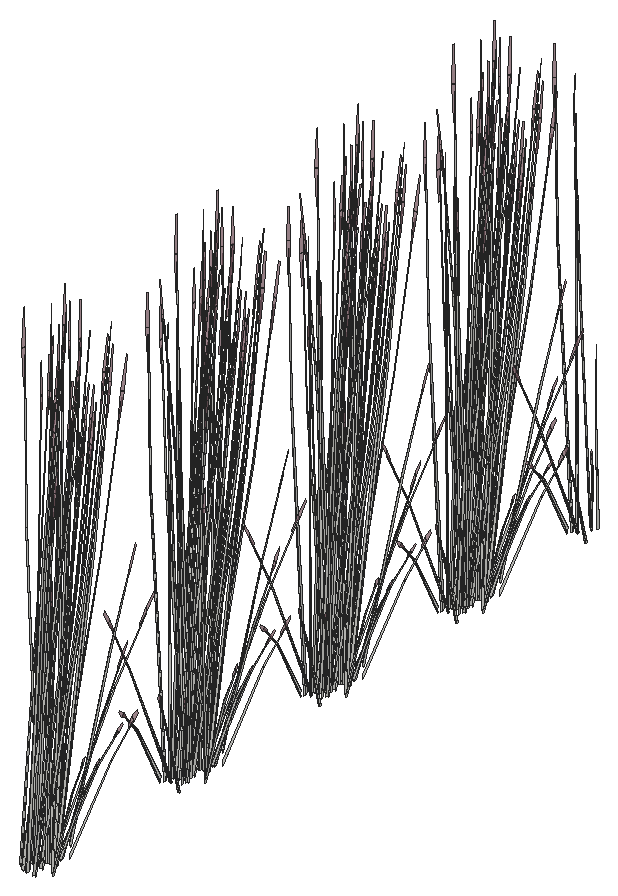
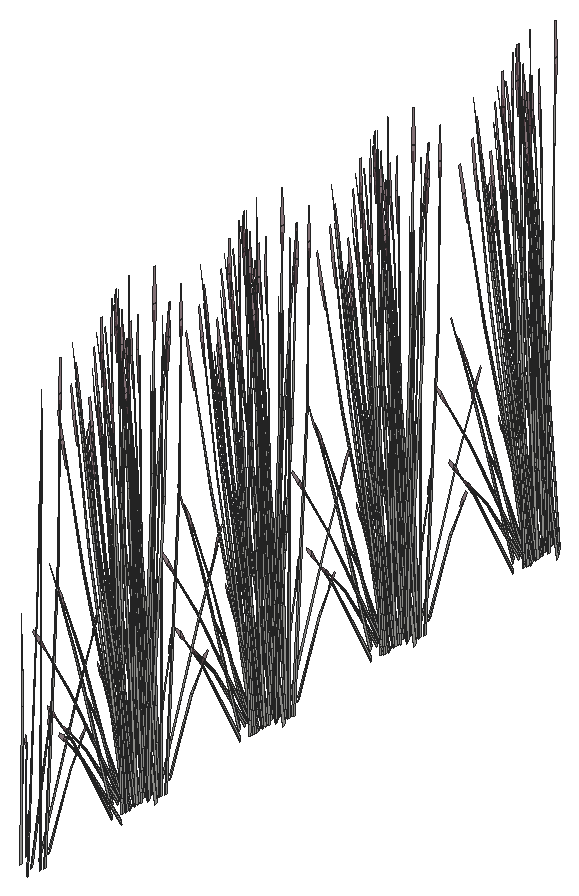
# SketchUp Ruby script. Lengths in inches.
U = 1.inch
M = Sketchup.active_model
def pt(a) = Geom::Point3d.new(a.map { |v| v * U })
def face(e, loops, mat)
  f = e.add_face(loops[0].map { |a| pt(a) })
  loops[1..].each { |l| e.add_face(l.map { |a| pt(a) }).erase! }
  f.material = f.back_material = mat if mat
  f
end
# faces: each face lists its corners as indices into pts; further lists are holes
def faces(e, pts, list, mat = nil) = list.each { |f| face(e, (f[0].is_a?(Array) ? f : [f]).map { |l| l.map { |i| pts[i] } }, mat) }
# xy, xz, yz: faces in a plane at the given z, y or x. An outline is a flat list of corners, or four numbers for a rectangle; further outlines are holes
def ring(l) = l.size == 4 ? [[l[0], l[1]], [l[2], l[1]], [l[2], l[3]], [l[0], l[3]]] : l.each_slice(2).to_a
def flat(e, list, mat, &to3) = list.each { |f| face(e, (f[0].is_a?(Array) ? f : [f]).map { |l| ring(l).map { |u, v| to3.(u, v) } }, mat) }
def xy(e, z, list, mat = nil) = flat(e, list, mat) { |x, y| [x, y, z] }
def xz(e, y, list, mat = nil) = flat(e, list, mat) { |x, z| [x, y, z] }
def yz(e, x, list, mat = nil) = flat(e, list, mat) { |y, z| [x, y, z] }
def lines(e, pts, list) = list.each { |a, b| e.add_line(pt(pts[a]), pt(pts[b])) }
# prism: a flat outline (further loops are holes) pulled along v
def prism(e, loops, v, mat = nil)
  f = face(e, loops, mat); d = Geom::Vector3d.new(v.map { |x| x * U })
  f.pushpull(f.normal.samedirection?(d) ? d.length : -d.length)
end
def box(e, o, s, mat = nil) = prism(e, [[o, [o[0] + s[0], o[1], o[2]], [o[0] + s[0], o[1] + s[1], o[2]], [o[0], o[1] + s[1], o[2]]]], [0, 0, s[2]], mat)
def at(x, y, z, deg = 0) = Geom::Transformation.translation(pt([x, y, z])) * Geom::Transformation.rotation(ORIGIN, Z_AXIS, deg.degrees)
def axes(o, x, y, z) = Geom::Transformation.new([*x, 0, *y, 0, *z, 0, *pt(o).to_a, 1])
def part(name) = M.definitions.add(name)
# library, detail: a bought-in or finely detailed component or shape, given as its bounding box
def library(name, o, s) = part(name).tap { |d| box(d.entities, o, s) }
def detail(e, o, s) = box(e.add_group.entities, o, s)
def put(e, d, t, mat = nil) = e.add_instance(d, t).tap { |i| i.material = mat if mat }
def group(e, t, mat = nil) = e.add_group.tap { |g| g.transformation = t; g.material = mat if mat }.entities
root = M.entities
M.materials.add("LightPink_Translucent").color = [144, 107, 117]
M.materials["LightPink_Translucent"].alpha = 0.75
c1 = part("blade")
p = [[2.15,0.21,22],[0,0.17,0],[0.09,0.45,0],[2.18,0.31,22],[2.29,0.31,22],[0.38,0.45,0],
  [2.48,0.24,33],[2.49,0.24,33],[2.48,0.22,33]]
faces(c1.entities,p,[[0,1,2,3],[4,5,2,3],[6,3,4,7],[8,0,3,6]])
c2 = part("seeds")
p = [[0.3,-0.1,1.38],[-0.01,-0.03,1.59],[-0.01,-0.03,0.03],[0.14,-0.07,-0.07],[0.29,-0.03,3],[0.15,0.01,3.11]]
faces(c2.entities,p,[[0,1,2,3],[1,0,4,5]],"LightPink_Translucent")
c3 = part("blade with seeds")
put(c3.entities,c1,at(0,0,0))
put(c3.entities,c2,axes([2.4,0.25,30.99],[1.5799,-0.05474,1.17369],[-0.12525,1.92788,0.29478],[-0.07173,-0.02425,1.56792]))
put(root,c3,axes([251.43,184.71,0.28],[0.04142,-0.03327,1.27986],[0.24917,0.18313,-0.19552],[0.00729,0.2064,0.218]))
put(root,c3,axes([252.07,132.79,0.8],[-0.12419,0.55096,-0.32471],[-0.25804,-0.26516,0.15627],[0,0.12701,1.04254]))
put(root,c3,axes([252.07,150.43,0.8],[-0.12419,0.55096,-0.32471],[-0.25804,-0.26516,0.15627],[0,0.12701,1.04254]))
put(root,c3,axes([252.07,166.7,0.8],[-0.12419,0.55096,-0.32471],[-0.25804,-0.26516,0.15627],[0,0.12701,1.04254]))
put(root,c3,axes([252.07,182.55,0.8],[-0.12419,0.55096,-0.32471],[-0.25804,-0.26516,0.15627],[0,0.12701,1.04254]))
put(root,c3,axes([252.5625,132.46,0.99],[-0.2011,-0.44539,0.12804],[0.20266,-0.432,0.25465],[-0.02221,0.09096,1.1642]))
put(root,c3,axes([252.5625,150.1,0.99],[-0.2011,-0.44539,0.12804],[0.20266,-0.432,0.25465],[-0.02221,0.09096,1.1642]))
put(root,c3,axes([252.5625,166.37,0.99],[-0.2011,-0.44539,0.12804],[0.20266,-0.432,0.25465],[-0.02221,0.09096,1.1642]))
put(root,c3,axes([252.5625,182.22,0.99],[-0.2011,-0.44539,0.12804],[0.20266,-0.432,0.25465],[-0.02221,0.09096,1.1642]))
put(root,c3,axes([251.87,132.2,0.79],[0,-0.70749,0],[0.32006,0,0],[0,0,1.30246]))
put(root,c3,axes([251.87,149.84,0.79],[0,-0.70749,0],[0.32006,0,0],[0,0,1.30246]))
put(root,c3,axes([251.87,166.11,0.79],[0,-0.70749,0],[0.32006,0,0],[0,0,1.30246]))
put(root,c3,axes([251.87,181.96,0.79],[0,-0.70749,0],[0.32006,0,0],[0,0,1.30246]))
put(root,c3,axes([251.57,149.97,0.96],[0.28839,0.29636,0.17466],[-0.1388,0.61578,0.36291],[0,-0.14195,1.16519]))
put(root,c3,axes([251.57,166.24,0.96],[0.28839,0.29636,0.17466],[-0.1388,0.61578,0.36291],[0,-0.14195,1.16519]))
put(root,c3,axes([251.57,182.09,0.96],[0.28839,0.29636,0.17466],[-0.1388,0.61578,0.36291],[0,-0.14195,1.16519]))
put(root,c3,axes([252.03,132.48,0.86],[0,0.70714,-0.04091],[-0.32006,0,0],[0,0.02222,1.30182]))
put(root,c3,axes([252.03,150.125,0.86],[0,0.70714,-0.04091],[-0.32006,0,0],[0,0.02222,1.30182]))
put(root,c3,axes([252.03,166.39,0.86],[0,0.70714,-0.04091],[-0.32006,0,0],[0,0.02222,1.30182]))
put(root,c3,axes([252.03,182.24,0.86],[0,0.70714,-0.04091],[-0.32006,0,0],[0,0.02222,1.30182]))
put(root,c3,axes([251.48,149.56,1.17],[-0.27795,0.03775,0.32471],[-0.02514,-0.62656,-0.15627],[0.04976,-0.0635,1.04254]))
put(root,c3,axes([251.48,165.83,1.17],[-0.27795,0.03775,0.32471],[-0.02514,-0.62656,-0.15627],[0.04976,-0.0635,1.04254]))
put(root,c3,axes([251.48,181.68,1.17],[-0.27795,0.03775,0.32471],[-0.02514,-0.62656,-0.15627],[0.04976,-0.0635,1.04254]))
put(root,c3,axes([251.35,130.84,0.99],[-0.07394,0.60768,0.12804],[-0.27057,-0.17197,0.25465],[0.04674,-0.00296,1.1642]))
put(root,c3,axes([251.35,148.48,0.99],[-0.07394,0.60768,0.12804],[-0.27057,-0.17197,0.25465],[0.04674,-0.00296,1.1642]))
put(root,c3,axes([251.35,164.75,0.99],[-0.07394,0.60768,0.12804],[-0.27057,-0.17197,0.25465],[0.04674,-0.00296,1.1642]))
put(root,c3,axes([251.35,180.6,0.99],[-0.07394,0.60768,0.12804],[-0.27057,-0.17197,0.25465],[0.04674,-0.00296,1.1642]))
put(root,c3,axes([251.875,133.85,0.86],[0.11128,0.70245,-0.04364],[-0.31797,0.24614,0],[0.00389,0.02453,1.2496]))
put(root,c3,axes([251.875,151.49,0.86],[0.11128,0.70245,-0.04364],[-0.31797,0.24614,0],[0.00389,0.02453,1.2496]))
put(root,c3,axes([251.875,167.76,0.86],[0.11128,0.70245,-0.04364],[-0.31797,0.24614,0],[0.00389,0.02453,1.2496]))
put(root,c3,axes([251.875,183.61,0.86],[0.11128,0.70245,-0.04364],[-0.31797,0.24614,0],[0.00389,0.02453,1.2496]))
put(root,c3,axes([251.21,147.73,0.91],[-0.16003,-0.61271,0],[0.26773,-0.34169,-0.37456],[0.06098,-0.07782,1.18819]))
put(root,c3,axes([251.21,164,0.91],[-0.16003,-0.61271,0],[0.26773,-0.34169,-0.37456],[0.06098,-0.07782,1.18819]))
put(root,c3,axes([251.21,179.85,0.91],[-0.16003,-0.61271,0],[0.26773,-0.34169,-0.37456],[0.06098,-0.07782,1.18819]))
put(root,c3,axes([251.21,194.84,0.91],[-0.16003,-0.61271,0],[0.26773,-0.34169,-0.37456],[0.06098,-0.07782,1.18819]))
put(root,c3,axes([252.79,132.93,0.79],[-0.3199,-0.00489,-0.03612],[0,-0.68339,0.36248],[-0.01005,0.15557,1.14929]))
put(root,c3,axes([252.79,150.57,0.79],[-0.3199,-0.00489,-0.03612],[0,-0.68339,0.36248],[-0.01005,0.15557,1.14929]))
put(root,c3,axes([252.79,166.84,0.79],[-0.3199,-0.00489,-0.03612],[0,-0.68339,0.36248],[-0.01005,0.15557,1.14929]))
put(root,c3,axes([252.79,182.69,0.79],[-0.3199,-0.00489,-0.03612],[0,-0.68339,0.36248],[-0.01005,0.15557,1.14929]))
put(root,c3,axes([252.16,130.87,0.99],[-0.27504,0.16229,0.12804],[-0.06792,-0.60396,0.25465],[0.02453,0.088,1.1642]))
put(root,c3,axes([252.16,148.51,0.99],[-0.27504,0.16229,0.12804],[-0.06792,-0.60396,0.25465],[0.02453,0.088,1.1642]))
put(root,c3,axes([252.16,164.78,0.99],[-0.27504,0.16229,0.12804],[-0.06792,-0.60396,0.25465],[0.02453,0.088,1.1642]))
put(root,c3,axes([252.16,180.64,0.99],[-0.27504,0.16229,0.12804],[-0.06792,-0.60396,0.25465],[0.02453,0.088,1.1642]))
put(root,c3,axes([251.88,146.25,1.2],[0.03283,0.35655,0.83364],[-0.18215,-0.19748,0.6125],[0.0196,-0.18257,0.18362]))
put(root,c3,axes([251.88,162.52,1.2],[0.03283,0.35655,0.83364],[-0.18215,-0.19748,0.6125],[0.0196,-0.18257,0.18362]))
put(root,c3,axes([251.88,178.37,1.2],[0.03283,0.35655,0.83364],[-0.18215,-0.19748,0.6125],[0.0196,-0.18257,0.18362]))
put(root,c3,axes([251.88,193.36,1.2],[0.03283,0.35655,0.83364],[-0.18215,-0.19748,0.6125],[0.0196,-0.18257,0.18362]))
put(root,c3,axes([251.71,131.75,0.91],[-0.21222,0.5549,0.33208],[-0.25213,-0.48983,0.13031],[0.05116,-0.05538,1.15295]))
put(root,c3,axes([251.71,149.39,0.91],[-0.21222,0.5549,0.33208],[-0.25213,-0.48983,0.13031],[0.05116,-0.05538,1.15295]))
put(root,c3,axes([251.71,165.66,0.91],[-0.21222,0.5549,0.33208],[-0.25213,-0.48983,0.13031],[0.05116,-0.05538,1.15295]))
put(root,c3,axes([251.71,181.52,0.91],[-0.21222,0.5549,0.33208],[-0.25213,-0.48983,0.13031],[0.05116,-0.05538,1.15295]))
put(root,c3,axes([252.08,132.63,0.8],[0.17867,0.39495,0],[-0.17867,0.39495,0],[0,0,1.22851]))
put(root,c3,axes([252.08,150.27,0.8],[0.17867,0.39495,0],[-0.17867,0.39495,0],[0,0,1.22851]))
put(root,c3,axes([252.08,166.54,0.8],[0.17867,0.39495,0],[-0.17867,0.39495,0],[0,0,1.22851]))
put(root,c3,axes([252.08,182.39,0.8],[0.17867,0.39495,0],[-0.17867,0.39495,0],[0,0,1.22851]))
put(root,c3,axes([252.07,132.17,1.17],[0.12419,-0.55096,0.32471],[0.25804,0.26516,-0.15627],[0,0.12701,1.04254]))
put(root,c3,axes([252.07,149.81,1.17],[0.12419,-0.55096,0.32471],[0.25804,0.26516,-0.15627],[0,0.12701,1.04254]))
put(root,c3,axes([252.07,166.08,1.17],[0.12419,-0.55096,0.32471],[0.25804,0.26516,-0.15627],[0,0.12701,1.04254]))
put(root,c3,axes([252.07,181.93,1.17],[0.12419,-0.55096,0.32471],[0.25804,0.26516,-0.15627],[0,0.12701,1.04254]))
put(root,c3,axes([251.97,134.08,0.79],[0.25804,0.27452,0],[-0.12419,0.5704,0],[0,0,1.26978]))
put(root,c3,axes([251.97,151.72,0.79],[0.25804,0.27452,0],[-0.12419,0.5704,0],[0,0,1.26978]))
put(root,c3,axes([251.97,167.99,0.79],[0.25804,0.27452,0],[-0.12419,0.5704,0],[0,0,1.26978]))
put(root,c3,axes([251.97,183.84,0.79],[0.25804,0.27452,0],[-0.12419,0.5704,0],[0,0,1.26978]))
put(root,c3,axes([251.99,132.03,0.92],[-0.32351,-0.12883,0.35707],[0.06584,-0.72759,0.14012],[0.04728,0.07026,1.23973]))
put(root,c3,axes([251.99,149.68,0.92],[-0.32351,-0.12883,0.35707],[0.06584,-0.72759,0.14012],[0.04728,0.07026,1.23973]))
put(root,c3,axes([251.99,165.95,0.92],[-0.32351,-0.12883,0.35707],[0.06584,-0.72759,0.14012],[0.04728,0.07026,1.23973]))
put(root,c3,axes([251.99,181.8,0.92],[-0.32351,-0.12883,0.35707],[0.06584,-0.72759,0.14012],[0.04728,0.07026,1.23973]))
put(root,c3,axes([252.73,133.03,0.66],[-0.17867,0.3815,-0.22483],[-0.17867,-0.3815,0.22483],[0,0.12288,1.00865]))
put(root,c3,axes([252.73,150.67,0.66],[-0.17867,0.3815,-0.22483],[-0.17867,-0.3815,0.22483],[0,0.12288,1.00865]))
put(root,c3,axes([252.73,166.9375,0.66],[-0.17867,0.3815,-0.22483],[-0.17867,-0.3815,0.22483],[0,0.12288,1.00865]))
put(root,c3,axes([252.73,182.79,0.66],[-0.17867,0.3815,-0.22483],[-0.17867,-0.3815,0.22483],[0,0.12288,1.00865]))
put(root,c3,axes([252.22,132.96,0.71],[0.09385,0.55983,-0.50233],[-0.27035,0.20162,-0.13184],[0.01037,0.18957,1.1088]))
put(root,c3,axes([252.22,150.6,0.71],[0.09385,0.55983,-0.50233],[-0.27035,0.20162,-0.13184],[0.01037,0.18957,1.1088]))
put(root,c3,axes([252.22,166.87,0.71],[0.09385,0.55983,-0.50233],[-0.27035,0.20162,-0.13184],[0.01037,0.18957,1.1088]))
put(root,c3,axes([252.22,182.72,0.71],[0.09385,0.55983,-0.50233],[-0.27035,0.20162,-0.13184],[0.01037,0.18957,1.1088]))
put(root,c3,axes([252.08,132.36,0.79],[0.28637,0,0],[0,0.63302,0],[0,0,1.29484]))
put(root,c3,axes([252.08,150,0.79],[0.28637,0,0],[0,0.63302,0],[0,0,1.29484]))
put(root,c3,axes([252.08,166.27,0.79],[0.28637,0,0],[0,0.63302,0],[0,0,1.29484]))
put(root,c3,axes([252.08,182.12,0.79],[0.28637,0,0],[0,0.63302,0],[0,0,1.29484]))
put(root,c3,axes([251.81,131.66,1.17],[-0.15376,-0.51322,0.32471],[0.2329,-0.3614,-0.15627],[0.04976,0.0635,1.04254]))
put(root,c3,axes([251.81,149.3,1.17],[-0.15376,-0.51322,0.32471],[0.2329,-0.3614,-0.15627],[0.04976,0.0635,1.04254]))
put(root,c3,axes([251.81,165.57,1.17],[-0.15376,-0.51322,0.32471],[0.2329,-0.3614,-0.15627],[0.04976,0.0635,1.04254]))
put(root,c3,axes([251.81,181.42,1.17],[-0.15376,-0.51322,0.32471],[0.2329,-0.3614,-0.15627],[0.04976,0.0635,1.04254]))
put(root,c3,axes([251.53,149.42,1.13],[-0.02983,-0.6977,-0.21117],[0.31064,-0.04219,-0.36291],[0.0547,-0.09294,1.15913]))
put(root,c3,axes([251.53,165.69,1.13],[-0.02983,-0.6977,-0.21117],[0.31064,-0.04219,-0.36291],[0.0547,-0.09294,1.15913]))
put(root,c3,axes([251.53,181.54,1.13],[-0.02983,-0.6977,-0.21117],[0.31064,-0.04219,-0.36291],[0.0547,-0.09294,1.15913]))
put(root,c3,axes([252.18,132.29,1.09],[0.23848,-0.17832,0.10509],[0.08351,0.5092,-0.30009],[0,0.11207,0.91989]))
put(root,c3,axes([252.18,149.93,1.09],[0.23848,-0.17832,0.10509],[0.08351,0.5092,-0.30009],[0,0.11207,0.91989]))
put(root,c3,axes([252.18,166.2,1.09],[0.23848,-0.17832,0.10509],[0.08351,0.5092,-0.30009],[0,0.11207,0.91989]))
put(root,c3,axes([252.18,182.05,1.09],[0.23848,-0.17832,0.10509],[0.08351,0.5092,-0.30009],[0,0.11207,0.91989]))
put(root,c3,axes([252.1,132.33,1.13],[0.28825,0.29175,-0.21117],[-0.1388,0.61578,-0.36291],[0.00906,0.15119,1.15913]))
put(root,c3,axes([252.1,149.98,1.13],[0.28825,0.29175,-0.21117],[-0.1388,0.61578,-0.36291],[0.00906,0.15119,1.15913]))
put(root,c3,axes([252.1,166.25,1.13],[0.28825,0.29175,-0.21117],[-0.1388,0.61578,-0.36291],[0.00906,0.15119,1.15913]))
put(root,c3,axes([252.1,182.1,1.13],[0.28825,0.29175,-0.21117],[-0.1388,0.61578,-0.36291],[0.00906,0.15119,1.15913]))
put(root,c3,axes([251.49,147.88,0.66],[0.23879,0.15129,-0.22483],[-0.06012,0.53279,0.22483],[0.04814,-0.06144,1.00865]))
put(root,c3,axes([251.49,164.15,0.66],[0.23879,0.15129,-0.22483],[-0.06012,0.53279,0.22483],[0.04814,-0.06144,1.00865]))
put(root,c3,axes([251.49,180,0.66],[0.23879,0.15129,-0.22483],[-0.06012,0.53279,0.22483],[0.04814,-0.06144,1.00865]))
put(root,c3,axes([252.15,147.24,1.07],[-0.07276,0.12376,1.03788],[-0.21789,-0.21662,-0.22321],[0.04039,-0.2694,0.44375]))
put(root,c3,axes([252.15,163.51,1.07],[-0.07276,0.12376,1.03788],[-0.21789,-0.21662,-0.22321],[0.04039,-0.2694,0.44375]))
put(root,c3,axes([252.15,179.36,1.07],[-0.07276,0.12376,1.03788],[-0.21789,-0.21662,-0.22321],[0.04039,-0.2694,0.44375]))
put(root,c3,axes([252.15,194.34,1.07],[-0.07276,0.12376,1.03788],[-0.21789,-0.21662,-0.22321],[0.04039,-0.2694,0.44375]))
put(root,c3,axes([252.73,132.47,0.99],[0,-0.61145,0.36036],[0.28637,0,0],[0,0.13926,1.14313]))
put(root,c3,axes([252.73,150.12,0.99],[0,-0.61145,0.36036],[0.28637,0,0],[0,0.13926,1.14313]))
put(root,c3,axes([252.73,166.38,0.99],[0,-0.61145,0.36036],[0.28637,0,0],[0,0.13926,1.14313]))
put(root,c3,axes([252.73,182.24,0.99],[0,-0.61145,0.36036],[0.28637,0,0],[0,0.13926,1.14313]))
put(root,c3,axes([252.85,133.04,0.66],[0,0.61145,-0.36036],[-0.28637,0,0],[0,0.13926,1.14313]))
put(root,c3,axes([252.85,150.68,0.66],[0,0.61145,-0.36036],[-0.28637,0,0],[0,0.13926,1.14313]))
put(root,c3,axes([252.85,166.95,0.66],[0,0.61145,-0.36036],[-0.28637,0,0],[0,0.13926,1.14313]))
put(root,c3,axes([252.85,182.8,0.66],[0,0.61145,-0.36036],[-0.28637,0,0],[0,0.13926,1.14313]))
put(root,c3,axes([251.43,147.64,0.66],[0.23955,-0.30573,-0.36036],[0.14318,0.54821,0],[0.05456,-0.06963,1.14313]))
put(root,c3,axes([251.43,163.91,0.66],[0.23955,-0.30573,-0.36036],[0.14318,0.54821,0],[0.05456,-0.06963,1.14313]))
put(root,c3,axes([251.43,179.76,0.66],[0.23955,-0.30573,-0.36036],[0.14318,0.54821,0],[0.05456,-0.06963,1.14313]))
put(root,c3,axes([251.43,194.74,0.66],[0.23955,-0.30573,-0.36036],[0.14318,0.54821,0],[0.05456,-0.06963,1.14313]))
put(root,c3,axes([251.91,131.51,1.09],[0.04938,-0.54569,0.10509],[0.24125,0.09472,-0.30009],[0.0439,0.05603,0.91989]))
put(root,c3,axes([251.91,149.16,1.09],[0.04938,-0.54569,0.10509],[0.24125,0.09472,-0.30009],[0.0439,0.05603,0.91989]))
put(root,c3,axes([251.91,165.43,1.09],[0.04938,-0.54569,0.10509],[0.24125,0.09472,-0.30009],[0.0439,0.05603,0.91989]))
put(root,c3,axes([251.91,181.28,1.09],[0.04938,-0.54569,0.10509],[0.24125,0.09472,-0.30009],[0.0439,0.05603,0.91989]))
put(root,c3,axes([252.25,130.5625,0.99],[-0.23955,-0.30573,0.36036],[0.14318,-0.54821,0],[0.05456,0.06963,1.14313]))
put(root,c3,axes([252.25,148.21,0.99],[-0.23955,-0.30573,0.36036],[0.14318,-0.54821,0],[0.05456,0.06963,1.14313]))
put(root,c3,axes([252.25,164.48,0.99],[-0.23955,-0.30573,0.36036],[0.14318,-0.54821,0],[0.05456,0.06963,1.14313]))
put(root,c3,axes([252.25,180.33,0.99],[-0.23955,-0.30573,0.36036],[0.14318,-0.54821,0],[0.05456,0.06963,1.14313]))
put(root,c3,axes([252.05,133.76,0.78],[0.26872,-0.20746,-0.13933],[0.09442,0.59762,0.00006],[0.02966,-0.02293,1.26212]))
put(root,c3,axes([252.05,151.4,0.78],[0.26872,-0.20746,-0.13933],[0.09442,0.59762,0.00006],[0.02966,-0.02293,1.26212]))
put(root,c3,axes([252.05,167.67,0.78],[0.26872,-0.20746,-0.13933],[0.09442,0.59762,0.00006],[0.02966,-0.02293,1.26212]))
put(root,c3,axes([252.05,183.52,0.78],[0.26872,-0.20746,-0.13933],[0.09442,0.59762,0.00006],[0.02966,-0.02293,1.26212]))
put(root,c3,axes([252.05,131.98,0.8],[0.15376,0.51322,-0.32471],[-0.2329,0.3614,0.15627],[0.04976,0.0635,1.04254]))
put(root,c3,axes([252.05,149.62,0.8],[0.15376,0.51322,-0.32471],[-0.2329,0.3614,0.15627],[0.04976,0.0635,1.04254]))
put(root,c3,axes([252.05,165.89,0.8],[0.15376,0.51322,-0.32471],[-0.2329,0.3614,0.15627],[0.04976,0.0635,1.04254]))
put(root,c3,axes([252.05,181.74,0.8],[0.15376,0.51322,-0.32471],[-0.2329,0.3614,0.15627],[0.04976,0.0635,1.04254]))
put(root,c3,axes([252.49,134.31,1.2],[-0.14411,-0.17581,0.83364],[0.18609,-0.17864,0.6125],[0.05019,0.15132,0.18362]))
put(root,c3,axes([252.49,151.95,1.2],[-0.14411,-0.17581,0.83364],[0.18609,-0.17864,0.6125],[0.05019,0.15132,0.18362]))
put(root,c3,axes([252.49,168.22,1.2],[-0.14411,-0.17581,0.83364],[0.18609,-0.17864,0.6125],[0.05019,0.15132,0.18362]))
put(root,c3,axes([252.49,184.07,1.2],[-0.14411,-0.17581,0.83364],[0.18609,-0.17864,0.6125],[0.05019,0.15132,0.18362]))
put(root,c3,axes([251.97,134.12,1.07],[0.00452,-0.20269,1.03788],[0.21585,-0.22641,-0.22321],[0.06663,0.2426,0.44375]))
put(root,c3,axes([251.97,151.76,1.07],[0.00452,-0.20269,1.03788],[0.21585,-0.22641,-0.22321],[0.06663,0.2426,0.44375]))
put(root,c3,axes([251.97,168.03,1.07],[0.00452,-0.20269,1.03788],[0.21585,-0.22641,-0.22321],[0.06663,0.2426,0.44375]))
put(root,c3,axes([251.97,183.88,1.07],[0.00452,-0.20269,1.03788],[0.21585,-0.22641,-0.22321],[0.06663,0.2426,0.44375]))
put(root,c3,axes([251.71,148.89,0.6875],[0.1724,-0.45959,-0.45255],[0.21416,0.41674,-0.11877],[0.06908,-0.11465,0.99892]))
put(root,c3,axes([251.71,165.16,0.6875],[0.1724,-0.45959,-0.45255],[0.21416,0.41674,-0.11877],[0.06908,-0.11465,0.99892]))
put(root,c3,axes([251.71,181.01,0.6875],[0.1724,-0.45959,-0.45255],[0.21416,0.41674,-0.11877],[0.06908,-0.11465,0.99892]))
put(root,c3,axes([251.71,196,0.6875],[0.1724,-0.45959,-0.45255],[0.21416,0.41674,-0.11877],[0.06908,-0.11465,0.99892]))
put(root,c3,axes([252.47,130.84,0.66],[0.06012,0.53279,-0.22483],[-0.23879,0.15129,0.22483],[0.04814,0.06144,1.00865]))
put(root,c3,axes([252.47,148.48,0.66],[0.06012,0.53279,-0.22483],[-0.23879,0.15129,0.22483],[0.04814,0.06144,1.00865]))
put(root,c3,axes([252.47,164.75,0.66],[0.06012,0.53279,-0.22483],[-0.23879,0.15129,0.22483],[0.04814,0.06144,1.00865]))
put(root,c3,axes([252.47,180.6,0.66],[0.06012,0.53279,-0.22483],[-0.23879,0.15129,0.22483],[0.04814,0.06144,1.00865]))
put(root,c3,axes([252.92,132.58,0.92],[0.32006,0,0],[0,0.68339,-0.37456],[0,0.15565,1.18819]))
put(root,c3,axes([252.92,150.22,0.92],[0.32006,0,0],[0,0.68339,-0.37456],[0,0.15565,1.18819]))
put(root,c3,axes([252.92,166.49,0.92],[0.32006,0,0],[0,0.68339,-0.37456],[0,0.15565,1.18819]))
put(root,c3,axes([252.92,182.34,0.92],[0.32006,0,0],[0,0.68339,-0.37456],[0,0.15565,1.18819]))
put(root,c3,axes([251.89,131.69,1.13],[0.25843,-0.40595,-0.21117],[0.17185,0.5736,-0.36291],[0.06376,0.05825,1.15913]))
put(root,c3,axes([251.89,149.33,1.13],[0.25843,-0.40595,-0.21117],[0.17185,0.5736,-0.36291],[0.06376,0.05825,1.15913]))
put(root,c3,axes([251.89,165.6,1.13],[0.25843,-0.40595,-0.21117],[0.17185,0.5736,-0.36291],[0.06376,0.05825,1.15913]))
put(root,c3,axes([251.89,181.45,1.13],[0.25843,-0.40595,-0.21117],[0.17185,0.5736,-0.36291],[0.06376,0.05825,1.15913]))
put(root,c3,axes([252.51,135.11,1.13],[-0.16414,-0.01918,0.76251],[0.10839,-0.40729,0.421],[0.06484,0.1447,0.59812]))
put(root,c3,axes([252.51,152.75,1.13],[-0.16414,-0.01918,0.76251],[0.10839,-0.40729,0.421],[0.06484,0.1447,0.59812]))
put(root,c3,axes([252.51,169.02,1.13],[-0.16414,-0.01918,0.76251],[0.10839,-0.40729,0.421],[0.06484,0.1447,0.59812]))
put(root,c3,axes([252.51,184.87,1.13],[-0.16414,-0.01918,0.76251],[0.10839,-0.40729,0.421],[0.06484,0.1447,0.59812]))
put(root,c3,axes([251.23,131.33,0.35],[-0.25194,0.2448,0.93574],[-0.08019,-0.7024,0.36359],[0.1547,0.01169,1.0643]))
put(root,c3,axes([251.23,148.97,0.35],[-0.25194,0.2448,0.93574],[-0.08019,-0.7024,0.36359],[0.1547,0.01169,1.0643]))
put(root,c3,axes([251.23,165.24,0.35],[-0.25194,0.2448,0.93574],[-0.08019,-0.7024,0.36359],[0.1547,0.01169,1.0643]))
put(root,c3,axes([251.23,181.09,0.35],[-0.25194,0.2448,0.93574],[-0.08019,-0.7024,0.36359],[0.1547,0.01169,1.0643]))
put(root,c3,axes([252.39,147.89,0.92],[0.16003,-0.61271,0],[0.26773,0.34169,-0.37456],[0.06098,0.07782,1.18819]))
put(root,c3,axes([252.39,164.16,0.92],[0.16003,-0.61271,0],[0.26773,0.34169,-0.37456],[0.06098,0.07782,1.18819]))
put(root,c3,axes([252.39,180.01,0.92],[0.16003,-0.61271,0],[0.26773,0.34169,-0.37456],[0.06098,0.07782,1.18819]))
put(root,c3,axes([252.66,147.62,0.28],[-0.03831,-0.04817,1.27986],[-0.0984,-0.53815,-0.19552],[0.06638,-0.14604,0.218]))
put(root,c3,axes([252.66,163.89,0.28],[-0.03831,-0.04817,1.27986],[-0.0984,-0.53815,-0.19552],[0.06638,-0.14604,0.218]))
put(root,c3,axes([252.66,179.74,0.28],[-0.03831,-0.04817,1.27986],[-0.0984,-0.53815,-0.19552],[0.06638,-0.14604,0.218]))
put(root,c3,axes([252.66,194.73,0.28],[-0.03831,-0.04817,1.27986],[-0.0984,-0.53815,-0.19552],[0.06638,-0.14604,0.218]))
put(root,c3,axes([252.54,130.61,0.66],[0.23955,0.30573,-0.36036],[-0.14318,0.54821,0],[0.05456,0.06963,1.14313]))
put(root,c3,axes([252.54,148.25,0.66],[0.23955,0.30573,-0.36036],[-0.14318,0.54821,0],[0.05456,0.06963,1.14313]))
put(root,c3,axes([252.54,164.52,0.66],[0.23955,0.30573,-0.36036],[-0.14318,0.54821,0],[0.05456,0.06963,1.14313]))
put(root,c3,axes([252.54,180.375,0.66],[0.23955,0.30573,-0.36036],[-0.14318,0.54821,0],[0.05456,0.06963,1.14313]))
put(root,c3,axes([252.53,134.96,0.28],[0.01865,-0.08828,1.27986],[0.23477,-0.25998,-0.19552],[0.07118,0.13456,0.218]))
put(root,c3,axes([252.53,152.6,0.28],[0.01865,-0.08828,1.27986],[0.23477,-0.25998,-0.19552],[0.07118,0.13456,0.218]))
put(root,c3,axes([252.53,168.875,0.28],[0.01865,-0.08828,1.27986],[0.23477,-0.25998,-0.19552],[0.07118,0.13456,0.218]))
put(root,c3,axes([252.53,184.73,0.28],[0.01865,-0.08828,1.27986],[0.23477,-0.25998,-0.19552],[0.07118,0.13456,0.218]))
put(root,c3,axes([252.1875,131.78,0.6875],[0.26625,0.10025,-0.45255],[-0.05619,0.61836,-0.11877],[0.07946,0.07493,0.99892]))
put(root,c3,axes([252.1875,149.43,0.6875],[0.26625,0.10025,-0.45255],[-0.05619,0.61836,-0.11877],[0.07946,0.07493,0.99892]))
put(root,c3,axes([252.1875,165.69,0.6875],[0.26625,0.10025,-0.45255],[-0.05619,0.61836,-0.11877],[0.07946,0.07493,0.99892]))
put(root,c3,axes([252.1875,181.55,0.6875],[0.26625,0.10025,-0.45255],[-0.05619,0.61836,-0.11877],[0.07946,0.07493,0.99892]))
put(root,c3,axes([253.32,132.15,0.83],[-0.15869,-0.39099,-0.04709],[0.1738,-0.35825,-0.21349],[0.04925,-0.02522,0.70419]))
put(root,c3,axes([253.32,149.79,0.83],[-0.15869,-0.39099,-0.04709],[0.1738,-0.35825,-0.21349],[0.04925,-0.02522,0.70419]))
put(root,c3,axes([253.32,166.06,0.83],[-0.15869,-0.39099,-0.04709],[0.1738,-0.35825,-0.21349],[0.04925,-0.02522,0.70419]))
put(root,c3,axes([253.32,181.91,0.83],[-0.15869,-0.39099,-0.04709],[0.1738,-0.35825,-0.21349],[0.04925,-0.02522,0.70419]))
put(root,c3,axes([252.96,147.8,1.2],[-0.08525,0.31126,0.83364],[-0.07328,-0.41819,0.6125],[0.07041,-0.10479,0.18362]))
put(root,c3,axes([252.96,164.07,1.2],[-0.08525,0.31126,0.83364],[-0.07328,-0.41819,0.6125],[0.07041,-0.10479,0.18362]))
put(root,c3,axes([252.96,179.92,1.2],[-0.08525,0.31126,0.83364],[-0.07328,-0.41819,0.6125],[0.07041,-0.10479,0.18362]))
put(root,c3,axes([252.96,194.91,1.2],[-0.08525,0.31126,0.83364],[-0.07328,-0.41819,0.6125],[0.07041,-0.10479,0.18362]))
put(root,c3,axes([253.36,132.86,1.2],[-0.15814,0.10094,0.83364],[0.07444,-0.41719,0.6125],[0.0839,0.02855,0.18362]))
put(root,c3,axes([253.36,150.51,1.2],[-0.15814,0.10094,0.83364],[0.07444,-0.41719,0.6125],[0.0839,0.02855,0.18362]))
put(root,c3,axes([253.36,166.78,1.2],[-0.15814,0.10094,0.83364],[0.07444,-0.41719,0.6125],[0.0839,0.02855,0.18362]))
put(root,c3,axes([253.36,182.625,1.2],[-0.15814,0.10094,0.83364],[0.07444,-0.41719,0.6125],[0.0839,0.02855,0.18362]))
put(root,c3,axes([252.85,148.69,1.07],[-0.09144,-0.01811,1.03788],[-0.09368,-0.48584,-0.22321],[0.11233,-0.13744,0.44375]))
put(root,c3,axes([252.85,164.96,1.07],[-0.09144,-0.01811,1.03788],[-0.09368,-0.48584,-0.22321],[0.11233,-0.13744,0.44375]))
put(root,c3,axes([252.85,180.8125,1.07],[-0.09144,-0.01811,1.03788],[-0.09368,-0.48584,-0.22321],[0.11233,-0.13744,0.44375]))
put(root,c3,axes([252.85,195.8,1.07],[-0.09144,-0.01811,1.03788],[-0.09368,-0.48584,-0.22321],[0.11233,-0.13744,0.44375]))
put(root,c3,axes([253.02,150.31,0.63],[-0.16485,0.07338,1.02759],[-0.02624,-0.58408,0.05882],[0.11546,-0.08841,0.58473]))
put(root,c3,axes([253.02,166.58,0.63],[-0.16485,0.07338,1.02759],[-0.02624,-0.58408,0.05882],[0.11546,-0.08841,0.58473]))
put(root,c3,axes([253.02,182.43,0.63],[-0.16485,0.07338,1.02759],[-0.02624,-0.58408,0.05882],[0.11546,-0.08841,0.58473]))
put(root,c3,axes([253.2,132.28,0.28],[-0.01338,-0.09283,1.27986],[0.09278,-0.54301,-0.19552],[0.09359,-0.00781,0.218]))
put(root,c3,axes([253.2,149.93,0.28],[-0.01338,-0.09283,1.27986],[0.09278,-0.54301,-0.19552],[0.09359,-0.00781,0.218]))
put(root,c3,axes([253.2,166.2,0.28],[-0.01338,-0.09283,1.27986],[0.09278,-0.54301,-0.19552],[0.09359,-0.00781,0.218]))
put(root,c3,axes([253.2,182.05,0.28],[-0.01338,-0.09283,1.27986],[0.09278,-0.54301,-0.19552],[0.09359,-0.00781,0.218]))
put(root,c3,axes([253.07,133.53,1.07],[-0.06164,-0.15038,1.03788],[0.0802,-0.49748,-0.22321],[0.12472,0.06739,0.44375]))
put(root,c3,axes([253.07,151.17,1.07],[-0.06164,-0.15038,1.03788],[0.0802,-0.49748,-0.22321],[0.12472,0.06739,0.44375]))
put(root,c3,axes([253.07,167.44,1.07],[-0.06164,-0.15038,1.03788],[0.0802,-0.49748,-0.22321],[0.12472,0.06739,0.44375]))
put(root,c3,axes([253.07,183.3,1.07],[-0.06164,-0.15038,1.03788],[0.0802,-0.49748,-0.22321],[0.12472,0.06739,0.44375]))
